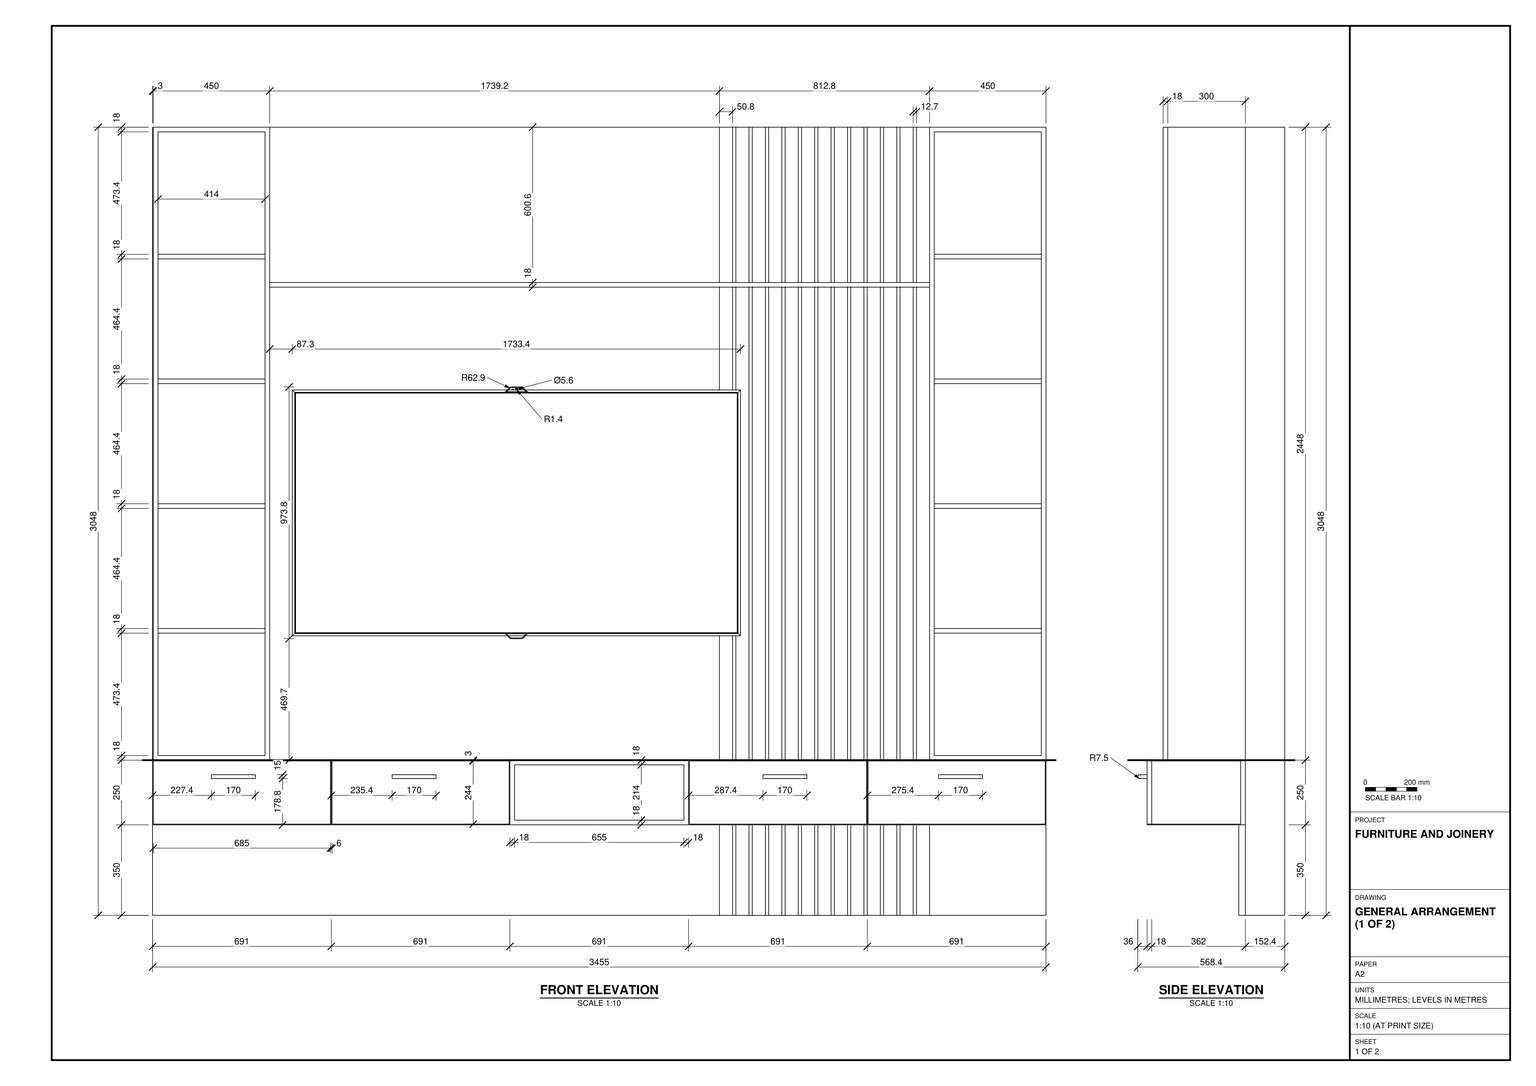
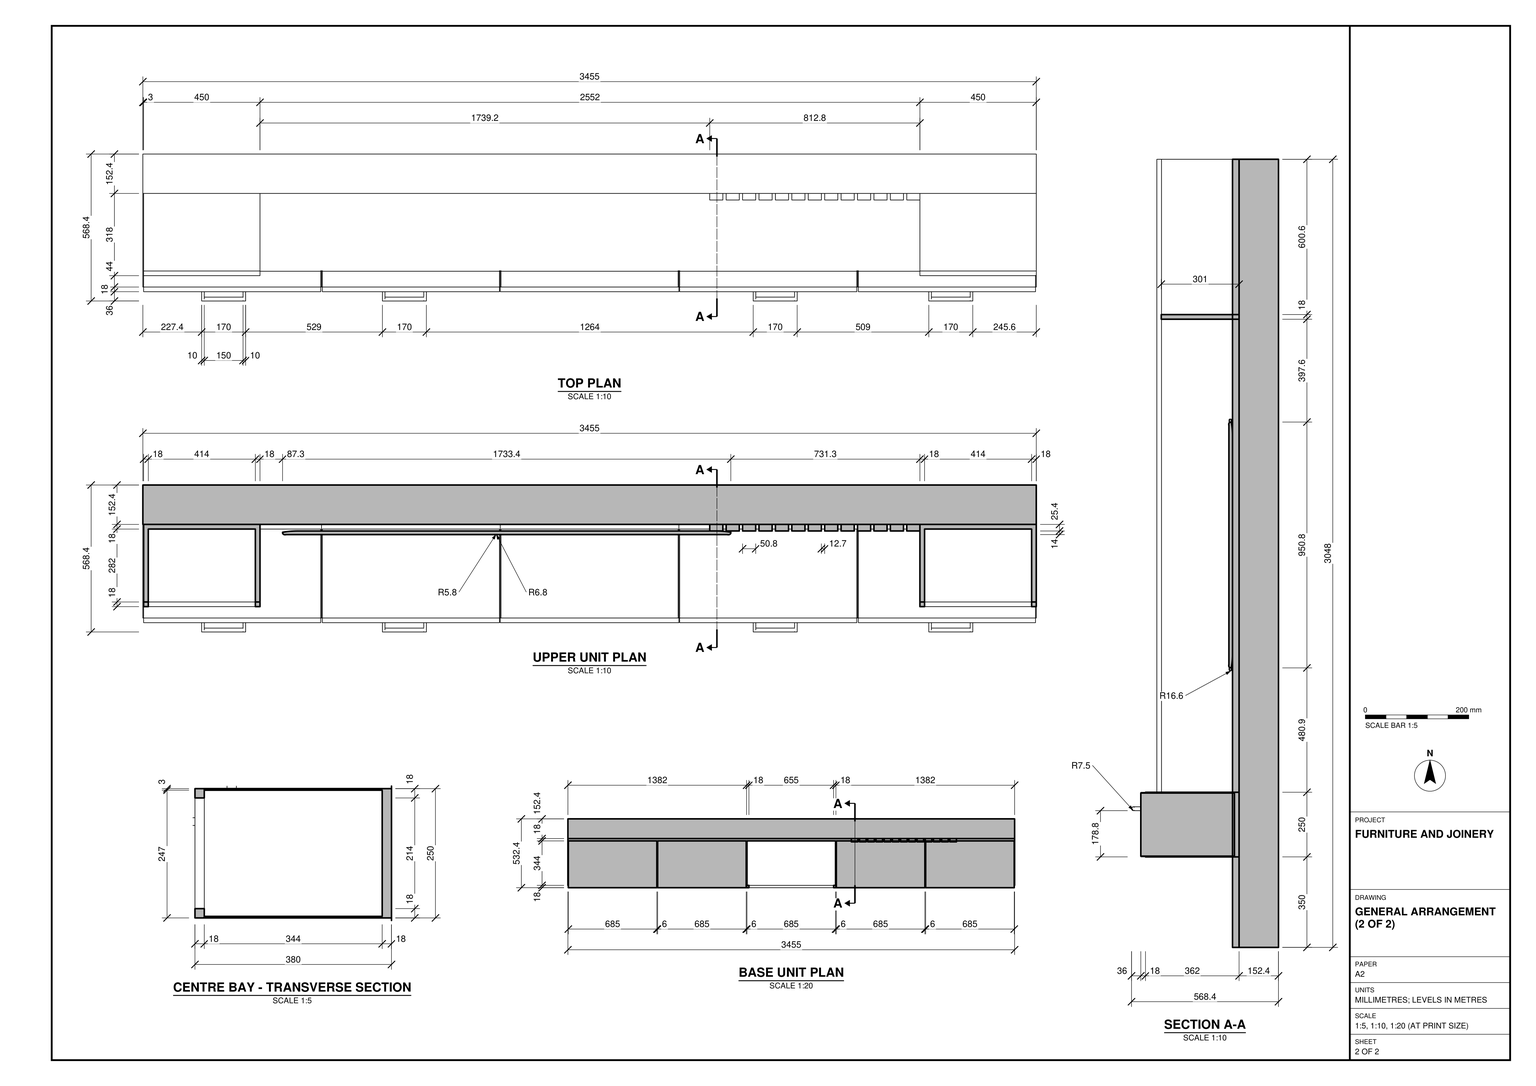
Build the television wall unit in SketchUp from task_files/diagram_01.pdf. Work in millimetres and use the floor as the 0 mm level. The complete assembly is 3455 mm wide, 568.4 mm deep from the back to the projecting pulls, and 3048 mm high. Model the full-height, 152.4 mm thick backing shown in plan and section.

Set the underside of the floating console 350 mm above the floor. Divide its 250 mm high body into five equal bays. Leave the middle bay open and fit a horizontal pull to each of the four closed fronts. Above the console, place a tall shelving unit at each end. Match their shelf heights and carry a single shelf across the space between the units. Use the plans and sections to set the shelving fronts back from the console fronts.

Place the television below the spanning shelf, close to the left shelving unit. Keep the backing plain to the left of the vertical slatted strip. Run the strip beside the right shelving unit and show its continuation below the console. Decor and loose items, including the television, may be represented by any suitable library component.

Keep the backing and each distinct joinery piece in separate groups or components, and use components for repeated parts. Save one SketchUp model as output_files/television_wall_unit_with_shelving_and_floating_console.skp.

# SketchUp Ruby script. Lengths in millimetres.
U = 1.mm
M = Sketchup.active_model
def pt(a) = Geom::Point3d.new(a.map { |v| v * U })
def face(e, loops, mat)
  f = e.add_face(loops[0].map { |a| pt(a) })
  loops[1..].each { |l| e.add_face(l.map { |a| pt(a) }).erase! }
  f.material = f.back_material = mat if mat
  f
end
# faces: each face lists its corners as indices into pts; further lists are holes
def faces(e, pts, list, mat = nil) = list.each { |f| face(e, (f[0].is_a?(Array) ? f : [f]).map { |l| l.map { |i| pts[i] } }, mat) }
# xy, xz, yz: faces in a plane at the given z, y or x. An outline is a flat list of corners, or four numbers for a rectangle; further outlines are holes
def ring(l) = l.size == 4 ? [[l[0], l[1]], [l[2], l[1]], [l[2], l[3]], [l[0], l[3]]] : l.each_slice(2).to_a
def flat(e, list, mat, &to3) = list.each { |f| face(e, (f[0].is_a?(Array) ? f : [f]).map { |l| ring(l).map { |u, v| to3.(u, v) } }, mat) }
def xy(e, z, list, mat = nil) = flat(e, list, mat) { |x, y| [x, y, z] }
def xz(e, y, list, mat = nil) = flat(e, list, mat) { |x, z| [x, y, z] }
def yz(e, x, list, mat = nil) = flat(e, list, mat) { |y, z| [x, y, z] }
def lines(e, pts, list) = list.each { |a, b| e.add_line(pt(pts[a]), pt(pts[b])) }
# prism: a flat outline (further loops are holes) pulled along v
def prism(e, loops, v, mat = nil)
  f = face(e, loops, mat); d = Geom::Vector3d.new(v.map { |x| x * U })
  f.pushpull(f.normal.samedirection?(d) ? d.length : -d.length)
end
def box(e, o, s, mat = nil) = prism(e, [[o, [o[0] + s[0], o[1], o[2]], [o[0] + s[0], o[1] + s[1], o[2]], [o[0], o[1] + s[1], o[2]]]], [0, 0, s[2]], mat)
def at(x, y, z, deg = 0) = Geom::Transformation.translation(pt([x, y, z])) * Geom::Transformation.rotation(ORIGIN, Z_AXIS, deg.degrees)
def axes(o, x, y, z) = Geom::Transformation.new([*x, 0, *y, 0, *z, 0, *pt(o).to_a, 1])
def part(name) = M.definitions.add(name)
# library, detail: a bought-in or finely detailed component or shape, given as its bounding box
def library(name, o, s) = part(name).tap { |d| box(d.entities, o, s) }
def detail(e, o, s) = box(e.add_group.entities, o, s)
def put(e, d, t, mat = nil) = e.add_instance(d, t).tap { |i| i.material = mat if mat }
def group(e, t, mat = nil) = e.add_group.tap { |g| g.transformation = t; g.material = mat if mat }.entities
root = M.entities
M.materials.add("0113 AP L161 ABSOLUTE WHITE").color = [243, 242, 236]
M.materials.add("0298 AP 719 GYPSY QUEEN").color = [205, 201, 209]
M.materials.add("[Wood Veneer 01]").color = [120, 70, 37]
c1 = part("Vertical wall slat")
box(c1.entities,[-50.8,-25.4,-3048],[50.8,25.4,3048],"[Wood Veneer 01]")
c2 = library("download?mid=50c7180b9fccec56d493bfe20f94b6ab&ctyp=sp&cv=p8.",[3795.5,1113.3,453.6],[1898.6,14.5,1067.8])
c3 = library("6-POIGNEE CLC2",[-85,-7.5,0],[170,15,36])
xy(root,2429.4,[[453,79,3005,380]],"[Wood Veneer 01]")
xy(root,2447.4,[[453,79,3005,380]],"[Wood Veneer 01]")
xz(root,79,[[453,2429.4,3005,2447.4]],"[Wood Veneer 01]")
xz(root,380,[[453,2429.4,3005,2447.4]])
yz(root,453,[[79,2429.4,380,2447.4]])
yz(root,3005,[[79,2429.4,380,2447.4]])
put(root,c1,at(3005,380,3048))
put(root,c1,at(2941.5,380,3048))
put(root,c1,at(2878,380,3048))
put(root,c1,at(2814.5,380,3048))
put(root,c1,at(2751,380,3048))
put(root,c1,at(2687.5,380,3048))
put(root,c1,at(2624,380,3048))
put(root,c1,at(2560.5,380,3048))
put(root,c1,at(2497,380,3048))
put(root,c1,at(2433.5,380,3048))
put(root,c1,at(2370,380,3048))
put(root,c1,at(2306.5,380,3048))
put(root,c1,at(2243,380,3048))
put(root,c2,axes([-2924.8,-773.2,656.1],[0.91296,0,0],[0,1,0],[0,0,0.91199]))
put(root,c3,axes([312.4,0,536.3],[1,0,0],[0,0,1],[0,-1,0]))
put(root,c3,axes([1011.4,0,536.3],[1,0,0],[0,0,1],[0,-1,0]))
put(root,c3,axes([2445.4,0,536.3],[1,0,0],[0,0,1],[0,-1,0]))
put(root,c3,axes([3124.4,0,536.3],[1,0,0],[0,0,1],[0,-1,0]))
g1 = group(root,at(0,380,0),"0298 AP 719 GYPSY QUEEN")
box(g1,[0,0,0],[3455,152.4,3048])
g2 = group(root,at(0,18,350),"[Wood Veneer 01]")
xy(g2,0,[[0,0,3455,362]])
xy(g2,3,[[3,0,688,344],[694,0,1379,344],[1385,0,2070,344],[2076,0,2761,344],[2767,0,3452,344]])
xy(g2,247,[[3,0,688,344],[694,0,1379,344],[1385,0,2070,344],[2076,0,2761,344],[2767,0,3452,344]])
xy(g2,250,[[0,0,691,362],[691,0,1382,362],[1382,0,2073,362],[2073,0,2764,362],[2764,0,3455,362]])
xz(g2,0,[[[0,0,691,250],[3,3,688,247]],[[691,0,1382,250],[694,3,1379,247]],[[1382,0,2073,250],[1385,3,2070,247]],[[2073,0,2764,250],[2076,3,2761,247]],[[2764,0,3455,250],[2767,3,3452,247]]])
xz(g2,344,[[3,3,688,247],[694,3,1379,247],[1385,3,2070,247],[2076,3,2761,247],[2767,3,3452,247]])
xz(g2,362,[[0,0,3455,250]])
yz(g2,0,[[0,0,362,250]])
yz(g2,3,[[0,3,344,247]])
yz(g2,688,[[0,3,344,247]])
yz(g2,694,[[0,3,344,247]])
yz(g2,1379,[[0,3,344,247]])
yz(g2,1385,[[0,3,344,247]])
yz(g2,2070,[[0,3,344,247]])
yz(g2,2076,[[0,3,344,247]])
yz(g2,2761,[[0,3,344,247]])
yz(g2,2767,[[0,3,344,247]])
yz(g2,3452,[[0,3,344,247]])
yz(g2,3455,[[0,0,362,250]])
g3 = group(root,at(0,18,350),"0113 AP L161 ABSOLUTE WHITE")
xy(g3,3,[[3,-18,688,0]],"0113 AP L161 ABSOLUTE WHITE")
xy(g3,247,[[3,-18,688,0]],"0113 AP L161 ABSOLUTE WHITE")
xz(g3,-18,[[3,3,688,247]],"0113 AP L161 ABSOLUTE WHITE")
xz(g3,0,[[[0,0,691,250],[3,3,688,247]]],"0113 AP L161 ABSOLUTE WHITE")
yz(g3,3,[[-18,3,0,247]],"0113 AP L161 ABSOLUTE WHITE")
yz(g3,688,[[-18,3,0,247]],"0113 AP L161 ABSOLUTE WHITE")
g4 = group(root,at(691,0,350),"0113 AP L161 ABSOLUTE WHITE")
xy(g4,3,[[3,0,688,18]])
xy(g4,247,[[3,0,688,18]])
xz(g4,0,[[3,3,688,247]])
xz(g4,18,[[[0,0,691,250],[3,3,688,247]]])
yz(g4,3,[[0,3,18,247]])
yz(g4,688,[[0,3,18,247]])
g5 = group(root,at(2073,0,350),"0113 AP L161 ABSOLUTE WHITE")
xy(g5,3,[[3,0,688,18]])
xy(g5,247,[[3,0,688,18]])
xz(g5,0,[[3,3,688,247]])
xz(g5,18,[[[0,0,691,250],[3,3,688,247]]])
yz(g5,3,[[0,3,18,247]])
yz(g5,688,[[0,3,18,247]])
g6 = group(root,at(3005,80,600),"[Wood Veneer 01]")
xy(g6,0,[[0,-18,450,0],[0,0,450,300]])
xy(g6,18,[[18,-18,432,0],[18,0,432,282]])
xy(g6,491.4,[[18,0,432,282]])
xy(g6,509.4,[[18,0,432,282]])
xy(g6,973.8,[[18,0,432,282]])
xy(g6,991.8,[[18,0,432,282]])
xy(g6,1456.2,[[18,0,432,282]])
xy(g6,1474.2,[[18,0,432,282]])
xy(g6,1938.6,[[18,0,432,282]])
xy(g6,1956.6,[[18,0,432,282]])
xy(g6,2430,[[18,-18,432,0],[18,0,432,282]])
xy(g6,2448,[[0,-18,450,0],[0,0,450,300]])
xz(g6,-18,[[[0,0,450,2448],[18,18,432,2430]]])
xz(g6,0,[[[0,0,450,2448],[18,18,432,2430]],[18,491.4,432,509.4],[18,973.8,432,991.8],[18,1456.2,432,1474.2],[18,1938.6,432,1956.6]])
xz(g6,282,[[18,18,432,491.4],[18,509.4,432,973.8],[18,991.8,432,1456.2],[18,1474.2,432,1938.6],[18,1956.6,432,2430]])
xz(g6,300,[[0,0,450,2448]])
yz(g6,0,[[-18,0,0,2448],[0,0,300,2448]])
yz(g6,18,[[-18,18,0,2430],[0,18,282,491.4],[0,509.4,282,973.8],[0,991.8,282,1456.2],[0,1474.2,282,1938.6],
  [0,1956.6,282,2430]])
yz(g6,432,[[-18,18,0,2430],[0,18,282,491.4],[0,509.4,282,973.8],[0,991.8,282,1456.2],[0,1474.2,282,1938.6],
  [0,1956.6,282,2430]])
yz(g6,450,[[-18,0,0,2448],[0,0,300,2448]])
g7 = group(root,at(3,80,600),"[Wood Veneer 01]")
xy(g7,0,[[0,-18,450,0],[0,0,450,300]])
xy(g7,18,[[18,-18,432,0],[18,0,432,282]])
xy(g7,491.4,[[18,0,432,282]])
xy(g7,509.4,[[18,0,432,282]])
xy(g7,973.8,[[18,0,432,282]])
xy(g7,991.8,[[18,0,432,282]])
xy(g7,1456.2,[[18,0,432,282]])
xy(g7,1474.2,[[18,0,432,282]])
xy(g7,1938.6,[[18,0,432,282]])
xy(g7,1956.6,[[18,0,432,282]])
xy(g7,2430,[[18,-18,432,0],[18,0,432,282]])
xy(g7,2448,[[0,-18,450,0],[0,0,450,300]])
xz(g7,-18,[[[0,0,450,2448],[18,18,432,2430]]])
xz(g7,0,[[[0,0,450,2448],[18,18,432,2430]],[18,491.4,432,509.4],[18,973.8,432,991.8],[18,1456.2,432,1474.2],[18,1938.6,432,1956.6]])
xz(g7,282,[[18,18,432,491.4],[18,509.4,432,973.8],[18,991.8,432,1456.2],[18,1474.2,432,1938.6],[18,1956.6,432,2430]])
xz(g7,300,[[0,0,450,2448]])
yz(g7,0,[[-18,0,0,2448],[0,0,300,2448]])
yz(g7,18,[[-18,18,0,2430],[0,18,282,491.4],[0,509.4,282,973.8],[0,991.8,282,1456.2],[0,1474.2,282,1938.6],
  [0,1956.6,282,2430]])
yz(g7,432,[[-18,18,0,2430],[0,18,282,491.4],[0,509.4,282,973.8],[0,991.8,282,1456.2],[0,1474.2,282,1938.6],
  [0,1956.6,282,2430]])
yz(g7,450,[[-18,0,0,2448],[0,0,300,2448]])
g8 = group(root,at(1382,18,350),"[Wood Veneer 01]")
prism(g8,[[[0,0,0],[0,0,250],[691,0,250],[691,0,0]],[[18,0,232],[18,0,18],[673,0,18],[673,0,232]]],[0,-18,0])
g9 = group(root,at(2764,0,350),"0113 AP L161 ABSOLUTE WHITE")
xy(g9,3,[[3,0,688,18]])
xy(g9,247,[[3,0,688,18]])
xz(g9,0,[[3,3,688,247]])
xz(g9,18,[[[0,0,691,250],[3,3,688,247]]])
yz(g9,3,[[0,3,18,247]])
yz(g9,688,[[0,3,18,247]])
